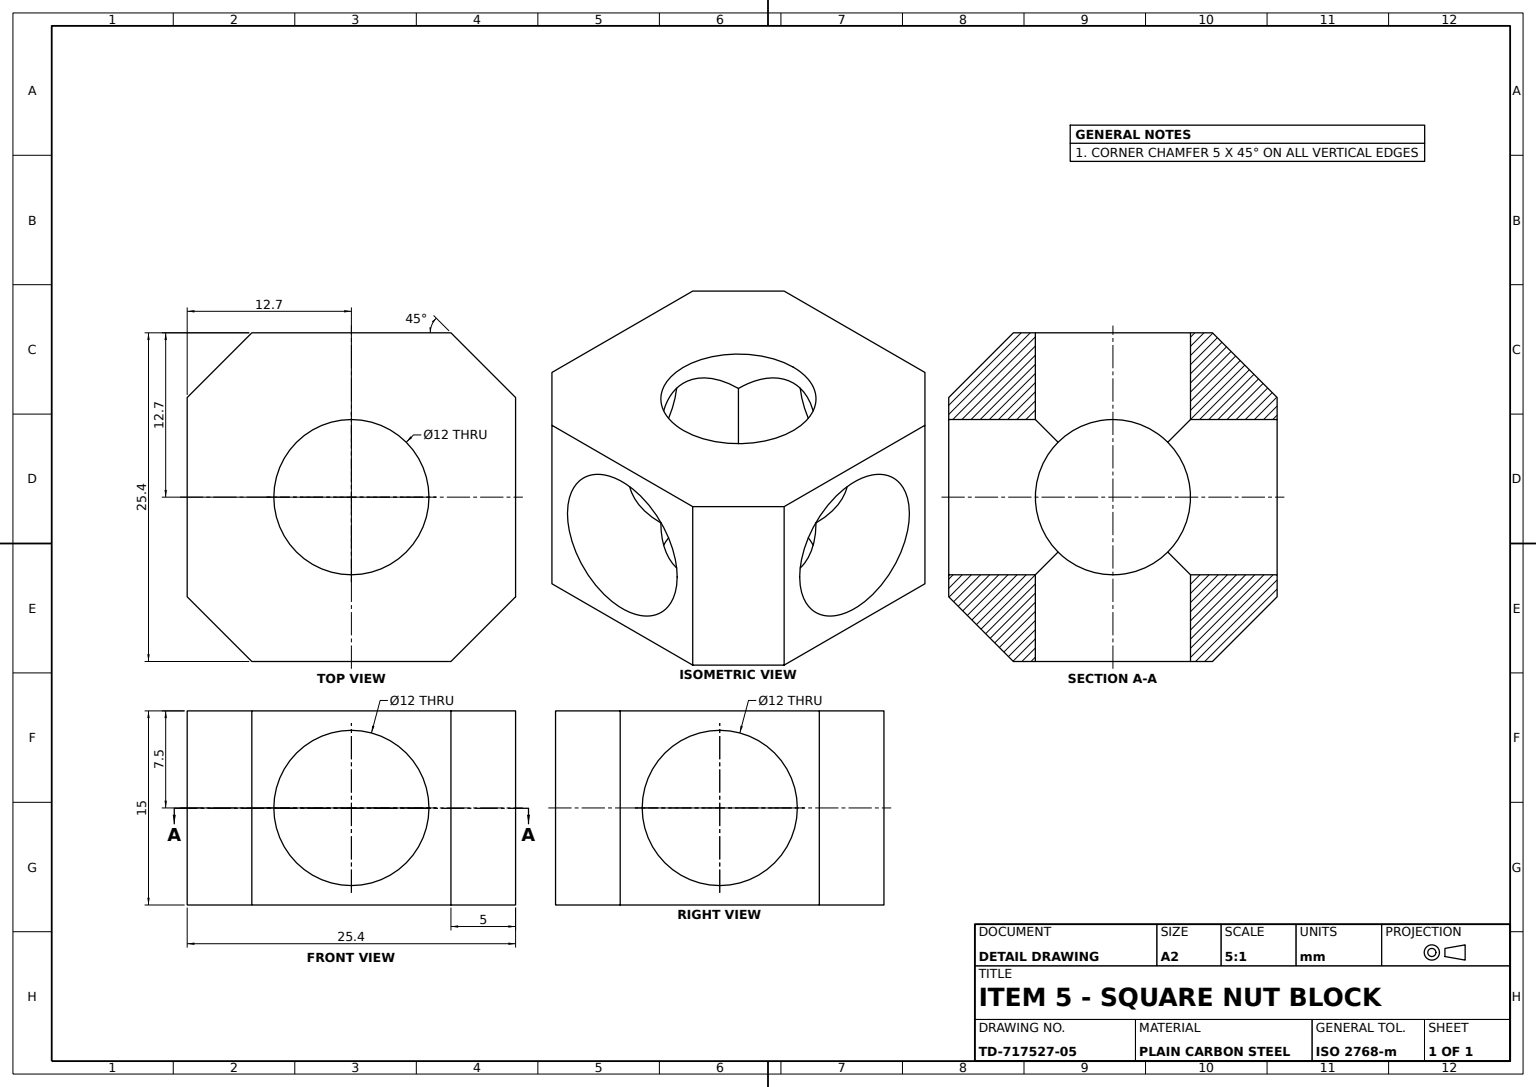
ISO-10303-21;
HEADER;
FILE_DESCRIPTION((''),'2;1');
FILE_NAME('','',(''),(''),'','','');
FILE_SCHEMA(('AUTOMOTIVE_DESIGN'));
ENDSEC;
DATA;
#1=APPLICATION_CONTEXT('');
#2=PRODUCT_CONTEXT('',#1,'mechanical');
#3=PRODUCT('','','',(#2));
#4=PRODUCT_DEFINITION_FORMATION('','',#3);
#5=PRODUCT_DEFINITION_CONTEXT('',#1,'design');
#6=PRODUCT_DEFINITION('','',#4,#5);
#7=PRODUCT_DEFINITION_SHAPE('','',#6);
#8=(LENGTH_UNIT()NAMED_UNIT(*)SI_UNIT(.MILLI.,.METRE.));
#9=(NAMED_UNIT(*)PLANE_ANGLE_UNIT()SI_UNIT($,.RADIAN.));
#10=(NAMED_UNIT(*)SI_UNIT($,.STERADIAN.)SOLID_ANGLE_UNIT());
#11=UNCERTAINTY_MEASURE_WITH_UNIT(LENGTH_MEASURE(1.E-05),#8,'distance_accuracy_value','');
#12=(GEOMETRIC_REPRESENTATION_CONTEXT(3)GLOBAL_UNCERTAINTY_ASSIGNED_CONTEXT((#11))GLOBAL_UNIT_ASSIGNED_CONTEXT((#8,#9,#10))REPRESENTATION_CONTEXT('',''));
#13=CARTESIAN_POINT('',(12.7,15.,-7.7));
#14=VERTEX_POINT('',#13);
#15=CARTESIAN_POINT('',(7.7,15.,-12.7));
#16=VERTEX_POINT('',#15);
#17=CARTESIAN_POINT('',(10.2,15.,-10.2));
#18=DIRECTION('',(-0.707106781,0.,-0.707106781));
#19=VECTOR('',#18,1000.);
#20=LINE('',#17,#19);
#21=EDGE_CURVE('',#14,#16,#20,.T.);
#22=ORIENTED_EDGE('',*,*,#21,.F.);
#23=CARTESIAN_POINT('',(12.7,0.,-7.7));
#24=VERTEX_POINT('',#23);
#25=DIRECTION('',(0.,1.,0.));
#26=VECTOR('',#25,1000.);
#27=LINE('',#13,#26);
#28=EDGE_CURVE('',#24,#14,#27,.T.);
#29=ORIENTED_EDGE('',*,*,#28,.F.);
#30=CARTESIAN_POINT('',(7.7,0.,-12.7));
#31=VERTEX_POINT('',#30);
#32=DIRECTION('',(0.707106781,0.,0.707106781));
#33=VECTOR('',#32,1000.);
#34=LINE('',#30,#33);
#35=EDGE_CURVE('',#31,#24,#34,.T.);
#36=ORIENTED_EDGE('',*,*,#35,.F.);
#37=DIRECTION('',(0.,-1.,0.));
#38=VECTOR('',#37,1000.);
#39=LINE('',#15,#38);
#40=EDGE_CURVE('',#16,#31,#39,.T.);
#41=ORIENTED_EDGE('',*,*,#40,.F.);
#42=EDGE_LOOP('',(#22,#29,#36,#41));
#43=FACE_OUTER_BOUND('',#42,.T.);
#44=DIRECTION('',(-0.707106781,0.,0.707106781));
#45=AXIS2_PLACEMENT_3D('',#15,#44,#37);
#46=PLANE('',#45);
#47=ADVANCED_FACE('',(#43),#46,.F.);
#48=CARTESIAN_POINT('',(12.7,15.,7.7));
#49=VERTEX_POINT('',#48);
#50=CARTESIAN_POINT('',(12.7,15.,12.7));
#51=DIRECTION('',(0.,0.,-1.));
#52=VECTOR('',#51,1000.);
#53=LINE('',#50,#52);
#54=EDGE_CURVE('',#49,#14,#53,.T.);
#55=ORIENTED_EDGE('',*,*,#54,.F.);
#56=CARTESIAN_POINT('',(12.7,0.,7.7));
#57=VERTEX_POINT('',#56);
#58=LINE('',#48,#38);
#59=EDGE_CURVE('',#49,#57,#58,.T.);
#60=ORIENTED_EDGE('',*,*,#59,.T.);
#61=CARTESIAN_POINT('',(12.7,0.,0.));
#62=LINE('',#61,#52);
#63=EDGE_CURVE('',#57,#24,#62,.T.);
#64=ORIENTED_EDGE('',*,*,#63,.T.);
#65=ORIENTED_EDGE('',*,*,#28,.T.);
#66=EDGE_LOOP('',(#55,#60,#64,#65));
#67=FACE_OUTER_BOUND('',#66,.T.);
#68=CARTESIAN_POINT('',(12.7,7.5,6.));
#69=VERTEX_POINT('',#68);
#70=CARTESIAN_POINT('',(12.7,7.5,-6.));
#71=VERTEX_POINT('',#70);
#72=CARTESIAN_POINT('',(12.7,7.5,0.));
#73=DIRECTION('',(1.,0.,0.));
#74=AXIS2_PLACEMENT_3D('',#72,#73,#51);
#75=CIRCLE('',#74,6.);
#76=EDGE_CURVE('',#69,#71,#75,.T.);
#77=ORIENTED_EDGE('',*,*,#76,.F.);
#78=EDGE_CURVE('',#71,#69,#75,.T.);
#79=ORIENTED_EDGE('',*,*,#78,.F.);
#80=EDGE_LOOP('',(#77,#79));
#81=FACE_BOUND('',#80,.T.);
#82=CARTESIAN_POINT('',(12.7,15.,0.));
#83=DIRECTION('',(-1.,0.,0.));
#84=DIRECTION('',(0.,0.,1.));
#85=AXIS2_PLACEMENT_3D('',#82,#83,#84);
#86=PLANE('',#85);
#87=ADVANCED_FACE('',(#67,#81),#86,.F.);
#88=CARTESIAN_POINT('',(0.,1.5,6.));
#89=VERTEX_POINT('',#88);
#90=CARTESIAN_POINT('',(-4.242641,3.257359,4.242641));
#91=VERTEX_POINT('',#90);
#92=CARTESIAN_POINT('',(-1.612567,1.5,6.));
#93=CARTESIAN_POINT('',(-3.102384,2.117103,5.382897));
#94=(BOUNDED_CURVE()B_SPLINE_CURVE(3,(#88,#92,#93,#90),.UNSPECIFIED.,.F.,.F.)B_SPLINE_CURVE_WITH_KNOTS((4,4),(3.141592654,3.926990817),.UNSPECIFIED.)CURVE()GEOMETRIC_REPRESENTATION_ITEM()RATIONAL_B_SPLINE_CURVE((1.,0.949253022,0.949253022,1.))REPRESENTATION_ITEM(''));
#95=EDGE_CURVE('',#89,#91,#94,.T.);
#96=ORIENTED_EDGE('',*,*,#95,.F.);
#97=CARTESIAN_POINT('',(0.,0.,6.));
#98=VERTEX_POINT('',#97);
#99=CARTESIAN_POINT('',(0.,-21.,6.));
#100=LINE('',#99,#26);
#101=EDGE_CURVE('',#98,#89,#100,.T.);
#102=ORIENTED_EDGE('',*,*,#101,.F.);
#103=CARTESIAN_POINT('',(0.,0.,-6.));
#104=VERTEX_POINT('',#103);
#105=CARTESIAN_POINT('',(0.,0.,0.));
#106=AXIS2_PLACEMENT_3D('',#105,#25,#84);
#107=CIRCLE('',#106,6.);
#108=EDGE_CURVE('',#104,#98,#107,.T.);
#109=ORIENTED_EDGE('',*,*,#108,.F.);
#110=CARTESIAN_POINT('',(0.,1.5,-6.));
#111=VERTEX_POINT('',#110);
#112=CARTESIAN_POINT('',(0.,-21.,-6.));
#113=LINE('',#112,#26);
#114=EDGE_CURVE('',#104,#111,#113,.T.);
#115=ORIENTED_EDGE('',*,*,#114,.T.);
#116=CARTESIAN_POINT('',(-4.242641,3.257359,-4.242641));
#117=VERTEX_POINT('',#116);
#118=CARTESIAN_POINT('',(-3.102384,2.117103,-5.382897));
#119=CARTESIAN_POINT('',(-1.612567,1.5,-6.));
#120=(BOUNDED_CURVE()B_SPLINE_CURVE(3,(#116,#118,#119,#110),.UNSPECIFIED.,.F.,.F.)B_SPLINE_CURVE_WITH_KNOTS((4,4),(5.497787144,6.283185307),.UNSPECIFIED.)CURVE()GEOMETRIC_REPRESENTATION_ITEM()RATIONAL_B_SPLINE_CURVE((1.,0.949253022,0.949253022,1.))REPRESENTATION_ITEM(''));
#121=EDGE_CURVE('',#117,#111,#120,.T.);
#122=ORIENTED_EDGE('',*,*,#121,.F.);
#123=CARTESIAN_POINT('',(-6.727922,0.772078,1.757359));
#124=CARTESIAN_POINT('',(-6.727922,0.772078,-1.757359));
#125=(BOUNDED_CURVE()B_SPLINE_CURVE(3,(#90,#123,#124,#116),.UNSPECIFIED.,.F.,.F.)B_SPLINE_CURVE_WITH_KNOTS((4,4),(2.35619449,3.926990817),.UNSPECIFIED.)CURVE()GEOMETRIC_REPRESENTATION_ITEM()RATIONAL_B_SPLINE_CURVE((1.,0.804737854,0.804737854,1.))REPRESENTATION_ITEM(''));
#126=EDGE_CURVE('',#91,#117,#125,.T.);
#127=ORIENTED_EDGE('',*,*,#126,.F.);
#128=EDGE_LOOP('',(#96,#102,#109,#115,#122,#127));
#129=FACE_OUTER_BOUND('',#128,.T.);
#130=CARTESIAN_POINT('',(0.,-21.,0.));
#131=AXIS2_PLACEMENT_3D('',#130,#25,#84);
#132=CYLINDRICAL_SURFACE('',#131,6.);
#133=ADVANCED_FACE('',(#129),#132,.F.);
#134=CARTESIAN_POINT('',(-6.,7.5,12.7));
#135=VERTEX_POINT('',#134);
#136=CARTESIAN_POINT('',(6.,7.5,12.7));
#137=VERTEX_POINT('',#136);
#138=CARTESIAN_POINT('',(0.,7.5,12.7));
#139=AXIS2_PLACEMENT_3D('',#138,#51,#83);
#140=CIRCLE('',#139,6.);
#141=EDGE_CURVE('',#135,#137,#140,.T.);
#142=ORIENTED_EDGE('',*,*,#141,.T.);
#143=EDGE_CURVE('',#137,#135,#140,.T.);
#144=ORIENTED_EDGE('',*,*,#143,.T.);
#145=EDGE_LOOP('',(#142,#144));
#146=FACE_BOUND('',#145,.T.);
#147=CARTESIAN_POINT('',(-7.7,15.,12.7));
#148=VERTEX_POINT('',#147);
#149=CARTESIAN_POINT('',(7.7,15.,12.7));
#150=VERTEX_POINT('',#149);
#151=CARTESIAN_POINT('',(-12.7,15.,12.7));
#152=VECTOR('',#73,1000.);
#153=LINE('',#151,#152);
#154=EDGE_CURVE('',#148,#150,#153,.T.);
#155=ORIENTED_EDGE('',*,*,#154,.F.);
#156=CARTESIAN_POINT('',(-7.7,0.,12.7));
#157=VERTEX_POINT('',#156);
#158=LINE('',#147,#38);
#159=EDGE_CURVE('',#148,#157,#158,.T.);
#160=ORIENTED_EDGE('',*,*,#159,.T.);
#161=CARTESIAN_POINT('',(7.7,0.,12.7));
#162=VERTEX_POINT('',#161);
#163=CARTESIAN_POINT('',(-12.7,0.,12.7));
#164=LINE('',#163,#152);
#165=EDGE_CURVE('',#157,#162,#164,.T.);
#166=ORIENTED_EDGE('',*,*,#165,.T.);
#167=LINE('',#149,#26);
#168=EDGE_CURVE('',#162,#150,#167,.T.);
#169=ORIENTED_EDGE('',*,*,#168,.T.);
#170=EDGE_LOOP('',(#155,#160,#166,#169));
#171=FACE_OUTER_BOUND('',#170,.T.);
#172=AXIS2_PLACEMENT_3D('',#151,#51,#83);
#173=PLANE('',#172);
#174=ADVANCED_FACE('',(#146,#171),#173,.F.);
#175=EDGE_CURVE('',#98,#104,#107,.T.);
#176=ORIENTED_EDGE('',*,*,#175,.F.);
#177=ORIENTED_EDGE('',*,*,#101,.T.);
#178=CARTESIAN_POINT('',(4.242641,3.257359,4.242641));
#179=VERTEX_POINT('',#178);
#180=CARTESIAN_POINT('',(3.102384,2.117103,5.382897));
#181=CARTESIAN_POINT('',(1.612567,1.5,6.));
#182=(BOUNDED_CURVE()B_SPLINE_CURVE(3,(#178,#180,#181,#88),.UNSPECIFIED.,.F.,.F.)B_SPLINE_CURVE_WITH_KNOTS((4,4),(2.35619449,3.141592654),.UNSPECIFIED.)CURVE()GEOMETRIC_REPRESENTATION_ITEM()RATIONAL_B_SPLINE_CURVE((1.,0.949253022,0.949253022,1.))REPRESENTATION_ITEM(''));
#183=EDGE_CURVE('',#179,#89,#182,.T.);
#184=ORIENTED_EDGE('',*,*,#183,.F.);
#185=CARTESIAN_POINT('',(4.242641,3.257359,-4.242641));
#186=VERTEX_POINT('',#185);
#187=CARTESIAN_POINT('',(6.727922,0.772078,-1.757359));
#188=CARTESIAN_POINT('',(6.727922,0.772078,1.757359));
#189=(BOUNDED_CURVE()B_SPLINE_CURVE(3,(#185,#187,#188,#178),.UNSPECIFIED.,.F.,.F.)B_SPLINE_CURVE_WITH_KNOTS((4,4),(5.497787144,7.068583471),.UNSPECIFIED.)CURVE()GEOMETRIC_REPRESENTATION_ITEM()RATIONAL_B_SPLINE_CURVE((1.,0.804737854,0.804737854,1.))REPRESENTATION_ITEM(''));
#190=EDGE_CURVE('',#186,#179,#189,.T.);
#191=ORIENTED_EDGE('',*,*,#190,.F.);
#192=CARTESIAN_POINT('',(1.612567,1.5,-6.));
#193=CARTESIAN_POINT('',(3.102384,2.117103,-5.382897));
#194=(BOUNDED_CURVE()B_SPLINE_CURVE(3,(#110,#192,#193,#185),.UNSPECIFIED.,.F.,.F.)B_SPLINE_CURVE_WITH_KNOTS((4,4),(0.,0.785398163),.UNSPECIFIED.)CURVE()GEOMETRIC_REPRESENTATION_ITEM()RATIONAL_B_SPLINE_CURVE((1.,0.949253022,0.949253022,1.))REPRESENTATION_ITEM(''));
#195=EDGE_CURVE('',#111,#186,#194,.T.);
#196=ORIENTED_EDGE('',*,*,#195,.F.);
#197=ORIENTED_EDGE('',*,*,#114,.F.);
#198=EDGE_LOOP('',(#176,#177,#184,#191,#196,#197));
#199=FACE_OUTER_BOUND('',#198,.T.);
#200=ADVANCED_FACE('',(#199),#132,.F.);
#201=CARTESIAN_POINT('',(-6.,7.5,-12.7));
#202=VERTEX_POINT('',#201);
#203=CARTESIAN_POINT('',(6.,7.5,-12.7));
#204=VERTEX_POINT('',#203);
#205=CARTESIAN_POINT('',(0.,7.5,-12.7));
#206=AXIS2_PLACEMENT_3D('',#205,#51,#83);
#207=CIRCLE('',#206,6.);
#208=EDGE_CURVE('',#202,#204,#207,.T.);
#209=ORIENTED_EDGE('',*,*,#208,.F.);
#210=EDGE_CURVE('',#204,#202,#207,.T.);
#211=ORIENTED_EDGE('',*,*,#210,.F.);
#212=EDGE_LOOP('',(#209,#211));
#213=FACE_BOUND('',#212,.T.);
#214=CARTESIAN_POINT('',(-7.7,0.,-12.7));
#215=VERTEX_POINT('',#214);
#216=CARTESIAN_POINT('',(-7.7,15.,-12.7));
#217=VERTEX_POINT('',#216);
#218=LINE('',#216,#26);
#219=EDGE_CURVE('',#215,#217,#218,.T.);
#220=ORIENTED_EDGE('',*,*,#219,.T.);
#221=CARTESIAN_POINT('',(12.7,15.,-12.7));
#222=VECTOR('',#83,1000.);
#223=LINE('',#221,#222);
#224=EDGE_CURVE('',#16,#217,#223,.T.);
#225=ORIENTED_EDGE('',*,*,#224,.F.);
#226=ORIENTED_EDGE('',*,*,#40,.T.);
#227=CARTESIAN_POINT('',(12.7,0.,-12.7));
#228=LINE('',#227,#222);
#229=EDGE_CURVE('',#31,#215,#228,.T.);
#230=ORIENTED_EDGE('',*,*,#229,.T.);
#231=EDGE_LOOP('',(#220,#225,#226,#230));
#232=FACE_OUTER_BOUND('',#231,.T.);
#233=AXIS2_PLACEMENT_3D('',#221,#84,#73);
#234=PLANE('',#233);
#235=ADVANCED_FACE('',(#213,#232),#234,.F.);
#236=CARTESIAN_POINT('',(-12.7,0.,7.7));
#237=VERTEX_POINT('',#236);
#238=CARTESIAN_POINT('',(-12.7,15.,7.7));
#239=VERTEX_POINT('',#238);
#240=LINE('',#238,#26);
#241=EDGE_CURVE('',#237,#239,#240,.T.);
#242=ORIENTED_EDGE('',*,*,#241,.F.);
#243=LINE('',#156,#19);
#244=EDGE_CURVE('',#157,#237,#243,.T.);
#245=ORIENTED_EDGE('',*,*,#244,.F.);
#246=ORIENTED_EDGE('',*,*,#159,.F.);
#247=CARTESIAN_POINT('',(-10.2,15.,10.2));
#248=LINE('',#247,#33);
#249=EDGE_CURVE('',#239,#148,#248,.T.);
#250=ORIENTED_EDGE('',*,*,#249,.F.);
#251=EDGE_LOOP('',(#242,#245,#246,#250));
#252=FACE_OUTER_BOUND('',#251,.T.);
#253=DIRECTION('',(0.707106781,0.,-0.707106781));
#254=AXIS2_PLACEMENT_3D('',#147,#253,#37);
#255=PLANE('',#254);
#256=ADVANCED_FACE('',(#252),#255,.F.);
#257=CARTESIAN_POINT('',(-12.7,7.5,6.));
#258=VERTEX_POINT('',#257);
#259=CARTESIAN_POINT('',(-6.,7.5,6.));
#260=VERTEX_POINT('',#259);
#261=CARTESIAN_POINT('',(-23.3,7.5,6.));
#262=LINE('',#261,#152);
#263=EDGE_CURVE('',#258,#260,#262,.T.);
#264=ORIENTED_EDGE('',*,*,#263,.F.);
#265=CARTESIAN_POINT('',(-12.7,7.5,-6.));
#266=VERTEX_POINT('',#265);
#267=CARTESIAN_POINT('',(-12.7,7.5,0.));
#268=AXIS2_PLACEMENT_3D('',#267,#73,#51);
#269=CIRCLE('',#268,6.);
#270=EDGE_CURVE('',#266,#258,#269,.T.);
#271=ORIENTED_EDGE('',*,*,#270,.F.);
#272=CARTESIAN_POINT('',(-6.,7.5,-6.));
#273=VERTEX_POINT('',#272);
#274=CARTESIAN_POINT('',(-23.3,7.5,-6.));
#275=LINE('',#274,#152);
#276=EDGE_CURVE('',#266,#273,#275,.T.);
#277=ORIENTED_EDGE('',*,*,#276,.T.);
#278=CARTESIAN_POINT('',(-4.242641,11.742641,-4.242641));
#279=VERTEX_POINT('',#278);
#280=CARTESIAN_POINT('',(-5.382897,10.602384,-5.382897));
#281=CARTESIAN_POINT('',(-6.,9.112567,-6.));
#282=(BOUNDED_CURVE()B_SPLINE_CURVE(3,(#278,#280,#281,#272),.UNSPECIFIED.,.F.,.F.)B_SPLINE_CURVE_WITH_KNOTS((4,4),(5.497787144,6.283185307),.UNSPECIFIED.)CURVE()GEOMETRIC_REPRESENTATION_ITEM()RATIONAL_B_SPLINE_CURVE((1.,0.949253022,0.949253022,1.))REPRESENTATION_ITEM(''));
#283=EDGE_CURVE('',#279,#273,#282,.T.);
#284=ORIENTED_EDGE('',*,*,#283,.F.);
#285=CARTESIAN_POINT('',(-4.242641,11.742641,4.242641));
#286=VERTEX_POINT('',#285);
#287=CARTESIAN_POINT('',(-6.727922,14.227922,-1.757359));
#288=CARTESIAN_POINT('',(-6.727922,14.227922,1.757359));
#289=(BOUNDED_CURVE()B_SPLINE_CURVE(3,(#278,#287,#288,#285),.UNSPECIFIED.,.F.,.T.)B_SPLINE_CURVE_WITH_KNOTS((4,4),(2.35619449,3.926990817),.UNSPECIFIED.)CURVE()GEOMETRIC_REPRESENTATION_ITEM()RATIONAL_B_SPLINE_CURVE((1.,0.804737854,0.804737854,1.))REPRESENTATION_ITEM(''));
#290=EDGE_CURVE('',#279,#286,#289,.T.);
#291=ORIENTED_EDGE('',*,*,#290,.T.);
#292=CARTESIAN_POINT('',(-6.,9.112567,6.));
#293=CARTESIAN_POINT('',(-5.382897,10.602384,5.382897));
#294=(BOUNDED_CURVE()B_SPLINE_CURVE(3,(#259,#292,#293,#285),.UNSPECIFIED.,.F.,.F.)B_SPLINE_CURVE_WITH_KNOTS((4,4),(3.141592654,3.926990817),.UNSPECIFIED.)CURVE()GEOMETRIC_REPRESENTATION_ITEM()RATIONAL_B_SPLINE_CURVE((1.,0.949253022,0.949253022,1.))REPRESENTATION_ITEM(''));
#295=EDGE_CURVE('',#260,#286,#294,.T.);
#296=ORIENTED_EDGE('',*,*,#295,.F.);
#297=EDGE_LOOP('',(#264,#271,#277,#284,#291,#296));
#298=FACE_OUTER_BOUND('',#297,.T.);
#299=CARTESIAN_POINT('',(-23.3,7.5,0.));
#300=AXIS2_PLACEMENT_3D('',#299,#73,#51);
#301=CYLINDRICAL_SURFACE('',#300,6.);
#302=ADVANCED_FACE('',(#298),#301,.F.);
#303=CARTESIAN_POINT('',(-6.,7.5,23.3));
#304=LINE('',#303,#52);
#305=EDGE_CURVE('',#135,#260,#304,.T.);
#306=ORIENTED_EDGE('',*,*,#305,.T.);
#307=ORIENTED_EDGE('',*,*,#295,.T.);
#308=CARTESIAN_POINT('',(0.,13.5,6.));
#309=VERTEX_POINT('',#308);
#310=CARTESIAN_POINT('',(-3.102384,12.882897,5.382897));
#311=CARTESIAN_POINT('',(-1.612567,13.5,6.));
#312=(BOUNDED_CURVE()B_SPLINE_CURVE(3,(#285,#310,#311,#308),.UNSPECIFIED.,.F.,.F.)B_SPLINE_CURVE_WITH_KNOTS((4,4),(2.35619449,3.141592654),.UNSPECIFIED.)CURVE()GEOMETRIC_REPRESENTATION_ITEM()RATIONAL_B_SPLINE_CURVE((1.,0.949253022,0.949253022,1.))REPRESENTATION_ITEM(''));
#313=EDGE_CURVE('',#286,#309,#312,.T.);
#314=ORIENTED_EDGE('',*,*,#313,.T.);
#315=CARTESIAN_POINT('',(4.242641,11.742641,4.242641));
#316=VERTEX_POINT('',#315);
#317=CARTESIAN_POINT('',(1.612567,13.5,6.));
#318=CARTESIAN_POINT('',(3.102384,12.882897,5.382897));
#319=(BOUNDED_CURVE()B_SPLINE_CURVE(3,(#308,#317,#318,#315),.UNSPECIFIED.,.F.,.T.)B_SPLINE_CURVE_WITH_KNOTS((4,4),(3.141592654,3.926990817),.UNSPECIFIED.)CURVE()GEOMETRIC_REPRESENTATION_ITEM()RATIONAL_B_SPLINE_CURVE((1.,0.949253022,0.949253022,1.))REPRESENTATION_ITEM(''));
#320=EDGE_CURVE('',#309,#316,#319,.T.);
#321=ORIENTED_EDGE('',*,*,#320,.T.);
#322=CARTESIAN_POINT('',(6.,7.5,6.));
#323=VERTEX_POINT('',#322);
#324=CARTESIAN_POINT('',(5.382897,10.602384,5.382897));
#325=CARTESIAN_POINT('',(6.,9.112567,6.));
#326=(BOUNDED_CURVE()B_SPLINE_CURVE(3,(#315,#324,#325,#322),.UNSPECIFIED.,.F.,.F.)B_SPLINE_CURVE_WITH_KNOTS((4,4),(2.35619449,3.141592654),.UNSPECIFIED.)CURVE()GEOMETRIC_REPRESENTATION_ITEM()RATIONAL_B_SPLINE_CURVE((1.,0.949253022,0.949253022,1.))REPRESENTATION_ITEM(''));
#327=EDGE_CURVE('',#316,#323,#326,.T.);
#328=ORIENTED_EDGE('',*,*,#327,.T.);
#329=CARTESIAN_POINT('',(6.,7.5,23.3));
#330=LINE('',#329,#52);
#331=EDGE_CURVE('',#137,#323,#330,.T.);
#332=ORIENTED_EDGE('',*,*,#331,.F.);
#333=ORIENTED_EDGE('',*,*,#141,.F.);
#334=EDGE_LOOP('',(#306,#307,#314,#321,#328,#332,#333));
#335=FACE_OUTER_BOUND('',#334,.T.);
#336=CARTESIAN_POINT('',(0.,7.5,23.3));
#337=AXIS2_PLACEMENT_3D('',#336,#51,#83);
#338=CYLINDRICAL_SURFACE('',#337,6.);
#339=ADVANCED_FACE('',(#335),#338,.F.);
#340=CARTESIAN_POINT('',(0.,15.,6.));
#341=VERTEX_POINT('',#340);
#342=CARTESIAN_POINT('',(0.,15.,-6.));
#343=VERTEX_POINT('',#342);
#344=CARTESIAN_POINT('',(0.,15.,0.));
#345=AXIS2_PLACEMENT_3D('',#344,#25,#84);
#346=CIRCLE('',#345,6.);
#347=EDGE_CURVE('',#341,#343,#346,.T.);
#348=ORIENTED_EDGE('',*,*,#347,.T.);
#349=CARTESIAN_POINT('',(0.,13.5,-6.));
#350=VERTEX_POINT('',#349);
#351=EDGE_CURVE('',#350,#343,#113,.T.);
#352=ORIENTED_EDGE('',*,*,#351,.F.);
#353=CARTESIAN_POINT('',(4.242641,11.742641,-4.242641));
#354=VERTEX_POINT('',#353);
#355=CARTESIAN_POINT('',(3.102384,12.882897,-5.382897));
#356=CARTESIAN_POINT('',(1.612567,13.5,-6.));
#357=(BOUNDED_CURVE()B_SPLINE_CURVE(3,(#353,#355,#356,#349),.UNSPECIFIED.,.F.,.F.)B_SPLINE_CURVE_WITH_KNOTS((4,4),(5.497787144,6.283185307),.UNSPECIFIED.)CURVE()GEOMETRIC_REPRESENTATION_ITEM()RATIONAL_B_SPLINE_CURVE((1.,0.949253022,0.949253022,1.))REPRESENTATION_ITEM(''));
#358=EDGE_CURVE('',#354,#350,#357,.T.);
#359=ORIENTED_EDGE('',*,*,#358,.F.);
#360=CARTESIAN_POINT('',(6.727922,14.227922,1.757359));
#361=CARTESIAN_POINT('',(6.727922,14.227922,-1.757359));
#362=(BOUNDED_CURVE()B_SPLINE_CURVE(3,(#315,#360,#361,#353),.UNSPECIFIED.,.F.,.F.)B_SPLINE_CURVE_WITH_KNOTS((4,4),(5.497787144,7.068583471),.UNSPECIFIED.)CURVE()GEOMETRIC_REPRESENTATION_ITEM()RATIONAL_B_SPLINE_CURVE((1.,0.804737854,0.804737854,1.))REPRESENTATION_ITEM(''));
#363=EDGE_CURVE('',#316,#354,#362,.T.);
#364=ORIENTED_EDGE('',*,*,#363,.F.);
#365=ORIENTED_EDGE('',*,*,#320,.F.);
#366=EDGE_CURVE('',#309,#341,#100,.T.);
#367=ORIENTED_EDGE('',*,*,#366,.T.);
#368=EDGE_LOOP('',(#348,#352,#359,#364,#365,#367));
#369=FACE_OUTER_BOUND('',#368,.T.);
#370=ADVANCED_FACE('',(#369),#132,.F.);
#371=ORIENTED_EDGE('',*,*,#358,.T.);
#372=CARTESIAN_POINT('',(-1.612567,13.5,-6.));
#373=CARTESIAN_POINT('',(-3.102384,12.882897,-5.382897));
#374=(BOUNDED_CURVE()B_SPLINE_CURVE(3,(#349,#372,#373,#278),.UNSPECIFIED.,.F.,.F.)B_SPLINE_CURVE_WITH_KNOTS((4,4),(0.,0.785398163),.UNSPECIFIED.)CURVE()GEOMETRIC_REPRESENTATION_ITEM()RATIONAL_B_SPLINE_CURVE((1.,0.949253022,0.949253022,1.))REPRESENTATION_ITEM(''));
#375=EDGE_CURVE('',#350,#279,#374,.T.);
#376=ORIENTED_EDGE('',*,*,#375,.T.);
#377=ORIENTED_EDGE('',*,*,#283,.T.);
#378=EDGE_CURVE('',#273,#202,#304,.T.);
#379=ORIENTED_EDGE('',*,*,#378,.T.);
#380=ORIENTED_EDGE('',*,*,#208,.T.);
#381=CARTESIAN_POINT('',(6.,7.5,-6.));
#382=VERTEX_POINT('',#381);
#383=EDGE_CURVE('',#382,#204,#330,.T.);
#384=ORIENTED_EDGE('',*,*,#383,.F.);
#385=CARTESIAN_POINT('',(6.,9.112567,-6.));
#386=CARTESIAN_POINT('',(5.382897,10.602384,-5.382897));
#387=(BOUNDED_CURVE()B_SPLINE_CURVE(3,(#381,#385,#386,#353),.UNSPECIFIED.,.F.,.T.)B_SPLINE_CURVE_WITH_KNOTS((4,4),(0.,0.785398163),.UNSPECIFIED.)CURVE()GEOMETRIC_REPRESENTATION_ITEM()RATIONAL_B_SPLINE_CURVE((1.,0.949253022,0.949253022,1.))REPRESENTATION_ITEM(''));
#388=EDGE_CURVE('',#382,#354,#387,.T.);
#389=ORIENTED_EDGE('',*,*,#388,.T.);
#390=EDGE_LOOP('',(#371,#376,#377,#379,#380,#384,#389));
#391=FACE_OUTER_BOUND('',#390,.T.);
#392=ADVANCED_FACE('',(#391),#338,.F.);
#393=EDGE_CURVE('',#258,#266,#269,.T.);
#394=ORIENTED_EDGE('',*,*,#393,.T.);
#395=ORIENTED_EDGE('',*,*,#270,.T.);
#396=EDGE_LOOP('',(#394,#395));
#397=FACE_BOUND('',#396,.T.);
#398=CARTESIAN_POINT('',(-12.7,15.,-7.7));
#399=VERTEX_POINT('',#398);
#400=CARTESIAN_POINT('',(-12.7,0.,-7.7));
#401=VERTEX_POINT('',#400);
#402=LINE('',#398,#38);
#403=EDGE_CURVE('',#399,#401,#402,.T.);
#404=ORIENTED_EDGE('',*,*,#403,.T.);
#405=CARTESIAN_POINT('',(-12.7,0.,-12.7));
#406=VECTOR('',#84,1000.);
#407=LINE('',#405,#406);
#408=EDGE_CURVE('',#401,#237,#407,.T.);
#409=ORIENTED_EDGE('',*,*,#408,.T.);
#410=ORIENTED_EDGE('',*,*,#241,.T.);
#411=CARTESIAN_POINT('',(-12.7,15.,-12.7));
#412=LINE('',#411,#406);
#413=EDGE_CURVE('',#399,#239,#412,.T.);
#414=ORIENTED_EDGE('',*,*,#413,.F.);
#415=EDGE_LOOP('',(#404,#409,#410,#414));
#416=FACE_OUTER_BOUND('',#415,.T.);
#417=AXIS2_PLACEMENT_3D('',#411,#73,#51);
#418=PLANE('',#417);
#419=ADVANCED_FACE('',(#397,#416),#418,.F.);
#420=VECTOR('',#44,1000.);
#421=LINE('',#56,#420);
#422=EDGE_CURVE('',#57,#162,#421,.T.);
#423=ORIENTED_EDGE('',*,*,#422,.F.);
#424=ORIENTED_EDGE('',*,*,#59,.F.);
#425=CARTESIAN_POINT('',(10.2,15.,10.2));
#426=VECTOR('',#253,1000.);
#427=LINE('',#425,#426);
#428=EDGE_CURVE('',#150,#49,#427,.T.);
#429=ORIENTED_EDGE('',*,*,#428,.F.);
#430=ORIENTED_EDGE('',*,*,#168,.F.);
#431=EDGE_LOOP('',(#423,#424,#429,#430));
#432=FACE_OUTER_BOUND('',#431,.T.);
#433=AXIS2_PLACEMENT_3D('',#48,#18,#37);
#434=PLANE('',#433);
#435=ADVANCED_FACE('',(#432),#434,.F.);
#436=ORIENTED_EDGE('',*,*,#95,.T.);
#437=CARTESIAN_POINT('',(-5.382897,4.397616,5.382897));
#438=CARTESIAN_POINT('',(-6.,5.887433,6.));
#439=(BOUNDED_CURVE()B_SPLINE_CURVE(3,(#90,#437,#438,#259),.UNSPECIFIED.,.F.,.F.)B_SPLINE_CURVE_WITH_KNOTS((4,4),(2.35619449,3.141592654),.UNSPECIFIED.)CURVE()GEOMETRIC_REPRESENTATION_ITEM()RATIONAL_B_SPLINE_CURVE((1.,0.949253022,0.949253022,1.))REPRESENTATION_ITEM(''));
#440=EDGE_CURVE('',#91,#260,#439,.T.);
#441=ORIENTED_EDGE('',*,*,#440,.T.);
#442=ORIENTED_EDGE('',*,*,#305,.F.);
#443=ORIENTED_EDGE('',*,*,#143,.F.);
#444=ORIENTED_EDGE('',*,*,#331,.T.);
#445=CARTESIAN_POINT('',(6.,5.887433,6.));
#446=CARTESIAN_POINT('',(5.382897,4.397616,5.382897));
#447=(BOUNDED_CURVE()B_SPLINE_CURVE(3,(#322,#445,#446,#178),.UNSPECIFIED.,.F.,.F.)B_SPLINE_CURVE_WITH_KNOTS((4,4),(3.141592654,3.926990817),.UNSPECIFIED.)CURVE()GEOMETRIC_REPRESENTATION_ITEM()RATIONAL_B_SPLINE_CURVE((1.,0.949253022,0.949253022,1.))REPRESENTATION_ITEM(''));
#448=EDGE_CURVE('',#323,#179,#447,.T.);
#449=ORIENTED_EDGE('',*,*,#448,.T.);
#450=ORIENTED_EDGE('',*,*,#183,.T.);
#451=EDGE_LOOP('',(#436,#441,#442,#443,#444,#449,#450));
#452=FACE_OUTER_BOUND('',#451,.T.);
#453=ADVANCED_FACE('',(#452),#338,.F.);
#454=ORIENTED_EDGE('',*,*,#422,.T.);
#455=ORIENTED_EDGE('',*,*,#165,.F.);
#456=ORIENTED_EDGE('',*,*,#244,.T.);
#457=ORIENTED_EDGE('',*,*,#408,.F.);
#458=LINE('',#400,#426);
#459=EDGE_CURVE('',#401,#215,#458,.T.);
#460=ORIENTED_EDGE('',*,*,#459,.T.);
#461=ORIENTED_EDGE('',*,*,#229,.F.);
#462=ORIENTED_EDGE('',*,*,#35,.T.);
#463=ORIENTED_EDGE('',*,*,#63,.F.);
#464=EDGE_LOOP('',(#454,#455,#456,#457,#460,#461,#462,#463));
#465=FACE_OUTER_BOUND('',#464,.T.);
#466=ORIENTED_EDGE('',*,*,#175,.T.);
#467=ORIENTED_EDGE('',*,*,#108,.T.);
#468=EDGE_LOOP('',(#466,#467));
#469=FACE_BOUND('',#468,.T.);
#470=PLANE('',#106);
#471=ADVANCED_FACE('',(#465,#469),#470,.F.);
#472=ORIENTED_EDGE('',*,*,#448,.F.);
#473=EDGE_CURVE('',#323,#69,#262,.T.);
#474=ORIENTED_EDGE('',*,*,#473,.T.);
#475=ORIENTED_EDGE('',*,*,#76,.T.);
#476=EDGE_CURVE('',#382,#71,#275,.T.);
#477=ORIENTED_EDGE('',*,*,#476,.F.);
#478=CARTESIAN_POINT('',(5.382897,4.397616,-5.382897));
#479=CARTESIAN_POINT('',(6.,5.887433,-6.));
#480=(BOUNDED_CURVE()B_SPLINE_CURVE(3,(#185,#478,#479,#381),.UNSPECIFIED.,.F.,.F.)B_SPLINE_CURVE_WITH_KNOTS((4,4),(5.497787144,6.283185307),.UNSPECIFIED.)CURVE()GEOMETRIC_REPRESENTATION_ITEM()RATIONAL_B_SPLINE_CURVE((1.,0.949253022,0.949253022,1.))REPRESENTATION_ITEM(''));
#481=EDGE_CURVE('',#186,#382,#480,.T.);
#482=ORIENTED_EDGE('',*,*,#481,.F.);
#483=ORIENTED_EDGE('',*,*,#190,.T.);
#484=EDGE_LOOP('',(#472,#474,#475,#477,#482,#483));
#485=FACE_OUTER_BOUND('',#484,.T.);
#486=ADVANCED_FACE('',(#485),#301,.F.);
#487=ORIENTED_EDGE('',*,*,#276,.F.);
#488=ORIENTED_EDGE('',*,*,#393,.F.);
#489=ORIENTED_EDGE('',*,*,#263,.T.);
#490=ORIENTED_EDGE('',*,*,#440,.F.);
#491=ORIENTED_EDGE('',*,*,#126,.T.);
#492=CARTESIAN_POINT('',(-6.,5.887433,-6.));
#493=CARTESIAN_POINT('',(-5.382897,4.397616,-5.382897));
#494=(BOUNDED_CURVE()B_SPLINE_CURVE(3,(#272,#492,#493,#116),.UNSPECIFIED.,.F.,.T.)B_SPLINE_CURVE_WITH_KNOTS((4,4),(0.,0.785398163),.UNSPECIFIED.)CURVE()GEOMETRIC_REPRESENTATION_ITEM()RATIONAL_B_SPLINE_CURVE((1.,0.949253022,0.949253022,1.))REPRESENTATION_ITEM(''));
#495=EDGE_CURVE('',#273,#117,#494,.T.);
#496=ORIENTED_EDGE('',*,*,#495,.F.);
#497=EDGE_LOOP('',(#487,#488,#489,#490,#491,#496));
#498=FACE_OUTER_BOUND('',#497,.T.);
#499=ADVANCED_FACE('',(#498),#301,.F.);
#500=ORIENTED_EDGE('',*,*,#403,.F.);
#501=CARTESIAN_POINT('',(-10.2,15.,-10.2));
#502=LINE('',#501,#420);
#503=EDGE_CURVE('',#217,#399,#502,.T.);
#504=ORIENTED_EDGE('',*,*,#503,.F.);
#505=ORIENTED_EDGE('',*,*,#219,.F.);
#506=ORIENTED_EDGE('',*,*,#459,.F.);
#507=EDGE_LOOP('',(#500,#504,#505,#506));
#508=FACE_OUTER_BOUND('',#507,.T.);
#509=AXIS2_PLACEMENT_3D('',#398,#32,#37);
#510=PLANE('',#509);
#511=ADVANCED_FACE('',(#508),#510,.F.);
#512=ORIENTED_EDGE('',*,*,#366,.F.);
#513=ORIENTED_EDGE('',*,*,#313,.F.);
#514=ORIENTED_EDGE('',*,*,#290,.F.);
#515=ORIENTED_EDGE('',*,*,#375,.F.);
#516=ORIENTED_EDGE('',*,*,#351,.T.);
#517=EDGE_CURVE('',#343,#341,#346,.T.);
#518=ORIENTED_EDGE('',*,*,#517,.T.);
#519=EDGE_LOOP('',(#512,#513,#514,#515,#516,#518));
#520=FACE_OUTER_BOUND('',#519,.T.);
#521=ADVANCED_FACE('',(#520),#132,.F.);
#522=ORIENTED_EDGE('',*,*,#495,.T.);
#523=ORIENTED_EDGE('',*,*,#121,.T.);
#524=ORIENTED_EDGE('',*,*,#195,.T.);
#525=ORIENTED_EDGE('',*,*,#481,.T.);
#526=ORIENTED_EDGE('',*,*,#383,.T.);
#527=ORIENTED_EDGE('',*,*,#210,.T.);
#528=ORIENTED_EDGE('',*,*,#378,.F.);
#529=EDGE_LOOP('',(#522,#523,#524,#525,#526,#527,#528));
#530=FACE_OUTER_BOUND('',#529,.T.);
#531=ADVANCED_FACE('',(#530),#338,.F.);
#532=ORIENTED_EDGE('',*,*,#363,.T.);
#533=ORIENTED_EDGE('',*,*,#388,.F.);
#534=ORIENTED_EDGE('',*,*,#476,.T.);
#535=ORIENTED_EDGE('',*,*,#78,.T.);
#536=ORIENTED_EDGE('',*,*,#473,.F.);
#537=ORIENTED_EDGE('',*,*,#327,.F.);
#538=EDGE_LOOP('',(#532,#533,#534,#535,#536,#537));
#539=FACE_OUTER_BOUND('',#538,.T.);
#540=ADVANCED_FACE('',(#539),#301,.F.);
#541=ORIENTED_EDGE('',*,*,#428,.T.);
#542=ORIENTED_EDGE('',*,*,#54,.T.);
#543=ORIENTED_EDGE('',*,*,#21,.T.);
#544=ORIENTED_EDGE('',*,*,#224,.T.);
#545=ORIENTED_EDGE('',*,*,#503,.T.);
#546=ORIENTED_EDGE('',*,*,#413,.T.);
#547=ORIENTED_EDGE('',*,*,#249,.T.);
#548=ORIENTED_EDGE('',*,*,#154,.T.);
#549=EDGE_LOOP('',(#541,#542,#543,#544,#545,#546,#547,#548));
#550=FACE_OUTER_BOUND('',#549,.T.);
#551=ORIENTED_EDGE('',*,*,#517,.F.);
#552=ORIENTED_EDGE('',*,*,#347,.F.);
#553=EDGE_LOOP('',(#551,#552));
#554=FACE_BOUND('',#553,.T.);
#555=PLANE('',#345);
#556=ADVANCED_FACE('',(#550,#554),#555,.T.);
#557=CLOSED_SHELL('',(#47,#87,#133,#174,#200,#235,#256,#302,#339,#370,#392,#419,#435,#453,#471,#486,#499,#511,#521,#531,#540,#556));
#558=MANIFOLD_SOLID_BREP('',#557);
#559=ADVANCED_BREP_SHAPE_REPRESENTATION('',(#558),#12);
#560=SHAPE_DEFINITION_REPRESENTATION(#7,#559);
ENDSEC;
END-ISO-10303-21;
